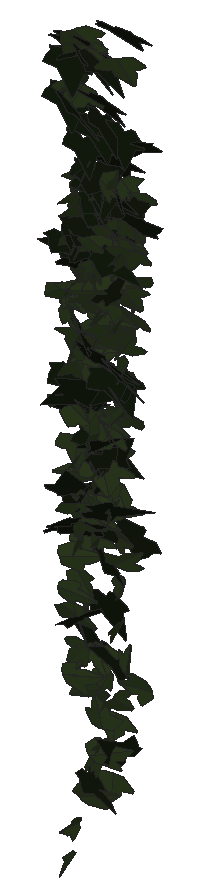
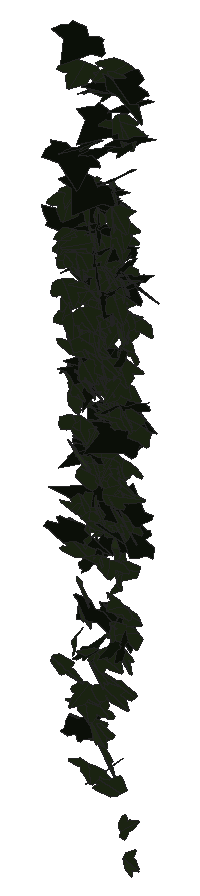
# SketchUp Ruby script. Lengths in millimetres.
U = 1.mm
M = Sketchup.active_model
def pt(a) = Geom::Point3d.new(a.map { |v| v * U })
def face(e, loops, mat)
  f = e.add_face(loops[0].map { |a| pt(a) })
  loops[1..].each { |l| e.add_face(l.map { |a| pt(a) }).erase! }
  f.material = f.back_material = mat if mat
  f
end
# faces: each face lists its corners as indices into pts; further lists are holes
def faces(e, pts, list, mat = nil) = list.each { |f| face(e, (f[0].is_a?(Array) ? f : [f]).map { |l| l.map { |i| pts[i] } }, mat) }
# xy, xz, yz: faces in a plane at the given z, y or x. An outline is a flat list of corners, or four numbers for a rectangle; further outlines are holes
def ring(l) = l.size == 4 ? [[l[0], l[1]], [l[2], l[1]], [l[2], l[3]], [l[0], l[3]]] : l.each_slice(2).to_a
def flat(e, list, mat, &to3) = list.each { |f| face(e, (f[0].is_a?(Array) ? f : [f]).map { |l| ring(l).map { |u, v| to3.(u, v) } }, mat) }
def xy(e, z, list, mat = nil) = flat(e, list, mat) { |x, y| [x, y, z] }
def xz(e, y, list, mat = nil) = flat(e, list, mat) { |x, z| [x, y, z] }
def yz(e, x, list, mat = nil) = flat(e, list, mat) { |y, z| [x, y, z] }
def lines(e, pts, list) = list.each { |a, b| e.add_line(pt(pts[a]), pt(pts[b])) }
# prism: a flat outline (further loops are holes) pulled along v
def prism(e, loops, v, mat = nil)
  f = face(e, loops, mat); d = Geom::Vector3d.new(v.map { |x| x * U })
  f.pushpull(f.normal.samedirection?(d) ? d.length : -d.length)
end
def box(e, o, s, mat = nil) = prism(e, [[o, [o[0] + s[0], o[1], o[2]], [o[0] + s[0], o[1] + s[1], o[2]], [o[0], o[1] + s[1], o[2]]]], [0, 0, s[2]], mat)
def at(x, y, z, deg = 0) = Geom::Transformation.translation(pt([x, y, z])) * Geom::Transformation.rotation(ORIGIN, Z_AXIS, deg.degrees)
def axes(o, x, y, z) = Geom::Transformation.new([*x, 0, *y, 0, *z, 0, *pt(o).to_a, 1])
def part(name) = M.definitions.add(name)
# library, detail: a bought-in or finely detailed component or shape, given as its bounding box
def library(name, o, s) = part(name).tap { |d| box(d.entities, o, s) }
def detail(e, o, s) = box(e.add_group.entities, o, s)
def put(e, d, t, mat = nil) = e.add_instance(d, t).tap { |i| i.material = mat if mat }
def group(e, t, mat = nil) = e.add_group.tap { |g| g.transformation = t; g.material = mat if mat }.entities
root = M.entities
M.materials.add("efeu1").color = [18, 25, 13]
M.materials.add("efeu2").color = [43, 57, 29]
c1 = part("ivyleaf_10")
p = [[0,12.8,-0.8],[-1.5,51.3,-10.9],[-4.9,51,-11.6],[-13.6,26.5,-7.3],[-13.2,15.9,-4.6],[-21.1,19.3,-7.2],
  [-29.5,16.3,-8.3],[-29.2,8.3,-6.2],[-19.7,-9.8,0.5],[-7.6,-13,4],[1,-12.2,5.8],[-0.4,51.1,-11.1],
  [-1.5,51.1,-10.9],[1,-12.4,5.9],[16.9,-12.4,3.5],[35.1,9.1,-5.1],[35,12.9,-6.1],[20.5,16.4,-4.9],
  [15.8,15,-3.8],[15.3,27.6,-7.1],[12.8,31.3,-7.8]]
faces(c1.entities,p,[[0,1,2,3,4,5,6,7,8,9,10],[11,12,0,13,14,15,16,17,18,19,20]],"efeu2")
c2 = part("ivyleaf_9")
p = [[39.1,54.8,31.7],[34.5,51.8,30.2],[-5.3,25.2,17.3],[-17.9,28.3,20.9],[-21.6,21.7,17],[-20.2,4.3,5.3],
  [-22.9,-0.3,2.5],[-17.1,-4,-0.6],[-2,-2.1,-1.2],[-0.7,-15.4,-10.1],[16.6,-22.3,-16.7],[21.1,-15.1,-12.5],
  [32.7,-10.7,-11],[46.1,-1.8,-6.6],[30.8,11.2,3.8]]
faces(c2.entities,p,[[0,1,2,3,4,5,6,7,8,9,10,11,12,13,14]],"efeu1")
put(root,c1,axes([1892.1,998.2,-11],[0.19463,-0.47894,0.44315],[0.19274,-0.43148,-0.48969],[1.2268,0.14377,0.00663]))
put(root,c1,axes([1890.9,1029.1,526.8],[0.05124,0.51211,-0.45605],[-0.09465,-0.45374,-0.51245],[-1.30166,0.05315,0.01931]))
put(root,c2,axes([1892.3,1001.6,639],[1.13233,0.14798,0.48713],[-0.90086,-0.11512,0.61309],[0.3568,-0.76028,0.00198]))
put(root,c1,axes([1879.9,1025.5,845.9],[0.7864,-0.38691,0.46588],[0.74396,-0.26036,-0.56292],[0.88029,0.56568,0.05956]))
put(root,c1,axes([1880.9,995,809.6],[-0.93857,-0.26754,-0.57621],[0.93865,0.29856,-0.56073],[0.76212,-0.6972,-0.019]))
put(root,c1,axes([1898.9,987.2,1003.2],[-0.90015,-0.5253,-0.05863],[0.07791,0.04204,-0.70684],[1.00293,-0.47473,0.00228]))
put(root,c2,axes([1884.6,1004,617.8],[-0.19577,0.57987,0.50112],[0.14823,-0.49509,0.58887],[1.45106,0.12881,0.00746]))
put(root,c1,axes([1893.1,1015.8,1002.9],[0.30987,-0.60948,0.3602],[0.28356,-0.33183,-0.62882],[1.31723,0.21481,0.05063]))
put(root,c2,axes([1923.4,990.5,1092.2],[-1.01779,0.459,0.33561],[-0.52931,0.1907,-0.70398],[-0.9439,-0.60187,0.03289]))
put(root,c1,axes([1884.2,986,1007.1],[-1.08831,-0.15728,-0.38861],[0.79191,-0.13262,-0.5586],[0.09749,-0.67855,0.19926]))
put(root,c1,axes([1901.7,1016.9,1052.5],[-0.44757,-0.68863,0.0359],[-0.02596,-0.03328,-0.72767],[1.31212,-0.23555,-0.00215]))
put(root,c1,axes([1920.8,1003.5,706.2],[-0.09636,0.0198,0.73075],[-1.32281,0.22566,-0.05427],[-0.43108,-0.69688,0.00319]))
put(root,c2,axes([1915.6,986.7,1442.6],[-0.21059,0.78295,0.17358],[-0.28841,0.15166,-0.78065],[-1.49879,-0.13919,0.12583]))
put(root,c1,axes([1914.2,1013,678.4],[-0.07211,-0.00104,0.71493],[-0.69492,-0.61549,-0.02024],[1.16981,-0.36569,0.03204]))
put(root,c1,axes([1877.9,1003.3,959.6],[0.47811,-0.17501,0.64405],[1.05261,-0.33057,-0.30556],[0.71094,0.60715,0.01928]))
put(root,c1,axes([1881.6,1004.1,426.4],[-0.83839,0.06542,-0.49262],[0.93221,-0.054,-0.44517],[-0.15971,-0.65865,-0.01243]))
put(root,c2,axes([1876,992.3,796.5],[0.92716,0.54428,-0.20873],[0.16349,0.20202,0.72728],[1.09732,-0.48998,0.068]))
put(root,c1,axes([1901.7,999.4,47.8],[-0.07165,0.02359,-0.66136],[-0.37794,-0.63231,-0.01125],[-1.20146,0.1975,0.04298]))
put(root,c1,axes([1900.5,997.6,1017.8],[0.06074,-0.68107,-0.2599],[0.06835,0.26131,-0.68033],[1.38569,0.01696,0.04495]))
put(root,c2,axes([1892.4,997.5,1352.9],[-0.51061,-0.73879,-0.08469],[0.06377,0.07793,-0.78599],[1.41385,-0.27033,0.00487]))
put(root,c1,axes([1910.2,1001.1,923.6],[-1.20894,-0.20678,0.21722],[-0.37356,-0.09804,-0.66731],[0.43155,-0.66413,0.03088]))
put(root,c1,axes([1896.5,1007.3,1095],[0.54539,-0.6458,0.24341],[0.22418,-0.21392,-0.70625],[1.29422,0.3092,0.01976]))
put(root,c2,axes([1880,1025.3,410.9],[0.27959,-0.07044,-0.76366],[1.27369,-0.36794,0.16268],[-0.71278,-0.68511,-0.00885]))
put(root,c2,axes([1891.5,994.4,1417.5],[-0.32094,-0.77685,-0.00116],[0.00042,0.00114,-0.79494],[1.47851,-0.16863,-0.00003]))
put(root,c2,axes([1882.8,970.1,588.7],[0.19865,0.77359,-0.37329],[0.09599,0.36987,0.7806],[1.63193,-0.11592,-0.00047]))
put(root,c2,axes([1888.9,1005.2,852],[-0.24132,-0.75891,-0.31784],[0.08183,0.31505,-0.76938],[1.56379,-0.1336,-0.00879]))
put(root,c2,axes([1882.7,996.5,1096.7],[0.13087,-0.62459,-0.43477],[0.27096,0.43939,-0.60871],[1.42278,-0.02623,0.15591]))
put(root,c2,axes([1893.7,996.8,1116],[0.51475,-0.39164,-0.60337],[-0.59231,0.51745,-0.47538],[1.23427,0.41165,0.02351]))
put(root,c1,axes([1907.4,1001.3,1008.6],[-0.60128,-0.56594,0.40793],[-0.0869,-0.43008,-0.63202],[1.32489,-0.28505,0.14368]))
put(root,c2,axes([1888.2,1009.6,1081.7],[0.21259,-0.69257,-0.31477],[-0.0378,0.31538,-0.70096],[1.44735,0.10996,0.02793]))
put(root,c1,axes([1877.9,1005,458.4],[-0.04579,-0.06446,-0.64016],[1.14648,-0.22727,0.00025],[-0.43011,-0.59894,0.06881]))
put(root,c1,axes([1875.1,1007.4,831],[0.66425,0.08698,-0.6989],[1.30234,0.14267,0.35948],[0.31714,-0.76806,-0.01237]))
put(root,c1,axes([1897.5,994.7,1102.9],[-0.49168,-0.51949,-0.50038],[0.53689,0.4164,-0.57795],[1.2634,-0.37912,0.05087]))
put(root,c1,axes([1900.6,1011,891.6],[-0.43543,-0.44557,-0.50735],[0.40774,0.4601,-0.50068],[1.21869,-0.31313,-0.01376]))
put(root,c1,axes([1908.8,1000,1090],[0.39131,-0.68349,-0.24067],[-0.05869,0.24169,-0.71274],[1.37786,0.20441,0.03799]))
put(root,c1,axes([1910.2,1006.8,1212.6],[-0.37225,-0.69304,0.2364],[-0.01059,-0.24328,-0.71779],[1.39357,-0.18697,0.05769]))
put(root,c1,axes([1887.2,1021.1,481.2],[0.86093,-0.12723,0.46148],[0.86001,-0.09607,-0.46943],[0.30069,0.63904,0.02131]))
put(root,c1,axes([1910.2,992.3,1180.1],[-0.38756,-0.71541,-0.11352],[0.02797,0.11382,-0.74364],[1.37832,-0.20347,-0.01683]))
put(root,c1,axes([1909.1,995.3,1381.4],[-0.23018,-0.78256,-0.05289],[0.10289,0.04507,-0.79048],[1.48921,-0.12407,0.04644]))
put(root,c2,axes([1889,1010.7,796.4],[1.33059,0.28438,0.2271],[0.39543,0.09191,-0.75473],[-0.56867,0.72932,0.00656]))
put(root,c1,axes([1912.2,992.3,1158.2],[-0.37361,-0.71421,-0.12632],[0.03883,0.12538,-0.74057],[1.37983,-0.19691,-0.01336]))
put(root,c1,axes([1911.3,992.9,715],[0.12809,-0.66352,-0.22259],[0.00896,0.22404,-0.66642],[1.33194,0.0623,0.02589]))
put(root,c2,axes([1926.3,992.2,838.1],[0.15156,0.15391,-0.78659],[-0.58079,-0.7251,-0.17277],[-1.41053,0.3151,-0.01338]))
put(root,c1,axes([1904.9,1006.3,994],[0.26511,0.60681,0.34219],[-0.06348,0.35438,-0.61484],[-1.32434,0.10449,0.09797]))
put(root,c1,axes([1910.8,990.7,567],[0.17328,-0.46133,-0.60617],[0.0576,0.61219,-0.46137],[1.44863,0.03084,0.09085]))
put(root,c1,axes([1912.9,998.6,572.7],[0.41058,-0.34624,0.53241],[-0.44883,0.47841,0.40669],[-1.12229,-0.318,0.03214]))
put(root,c1,axes([1895.1,1006.7,634.5],[-0.88033,0.32518,-0.48346],[0.7346,-0.29139,-0.56528],[-0.83066,-0.60231,0.01246]))
put(root,c1,axes([1906.3,994.6,876.2],[-0.62994,-0.60809,-0.42999],[0.44353,0.36234,-0.69182],[1.34625,-0.40392,0.02672]))
put(root,c1,axes([1911.9,992.5,1368.5],[1.45429,0.12089,-0.18392],[-0.37101,0.06325,-0.76833],[-0.19447,0.7834,0.09042]))
put(root,c1,axes([1917.3,981.8,914.1],[-0.06072,0.07864,0.80259],[-0.60761,0.73636,-0.08484],[-1.40941,-0.32084,0.002]))
put(root,c2,axes([1890.5,991.8,1344.7],[0.7805,-0.68862,0.00741],[0.02242,-0.00161,-0.80143],[1.31046,0.41016,0.0093]))
put(root,c1,axes([1901,1026.6,432.3],[-0.09377,-0.05383,0.68033],[0.67338,-0.58529,-0.02069],[1.11067,0.35031,0.06998]))
put(root,c1,axes([1886.1,1020.6,837.8],[0.52865,-0.05979,0.6487],[1.23953,0.00986,-0.27797],[0.02748,0.7056,0.05885]))
put(root,c1,axes([1902.1,993.1,736.4],[1.3072,-0.18781,0.22299],[0.4078,-0.06181,-0.71205],[0.37626,0.71948,-0.00296]))
put(root,c2,axes([1885.5,987.4,1455],[1.38474,-0.07712,0.3361],[0.64382,0.00739,-0.73062],[0.12731,0.80143,0.03908]))
put(root,c1,axes([1919.8,987.3,376.6],[0.96125,-0.49047,-0.24955],[-0.30952,0.19055,-0.70369],[1.00056,0.53015,0.02206]))
put(root,c1,axes([1888.9,1003.2,311.2],[0.55941,-0.25205,-0.63911],[1.1567,-0.22872,0.36972],[-0.60964,-0.66524,0.11504]))
put(root,c2,axes([1901.2,1014.7,401.5],[0.87533,-0.56043,-0.25866],[-0.29392,0.20783,-0.7249],[1.13738,0.48502,0.01174]))
put(root,c1,axes([1924,1002.8,639.9],[0.91718,-0.57651,-0.34397],[-0.42094,0.26343,-0.7514],[1.20633,0.53025,-0.00068]))
put(root,c1,axes([1920.5,1000,1035.6],[0.18194,-0.43647,-0.55522],[-0.08957,0.5551,-0.44448],[1.34114,0.09629,0.04564]))
put(root,c2,axes([1926.6,977.9,439.8],[0.09141,0.80891,-0.11699],[-0.01363,-0.11677,-0.81033],[-1.55547,0.04856,0.00023]))
put(root,c1,axes([1930.1,992,1042.8],[-1.08717,0.24738,0.35267],[-0.65261,0.09344,-0.62094],[-0.49627,-0.6648,0.04395]))
put(root,c1,axes([1936.4,1003.7,301.4],[-0.82061,-0.12625,0.49892],[-0.8843,-0.18438,-0.4482],[0.42116,-0.63312,0.03104]))
put(root,c1,axes([1912.4,988.8,624.2],[-1.18125,-0.27224,-0.27051],[0.48408,0.09338,-0.67757],[0.54698,-0.67058,0.01547]))
put(root,c1,axes([1912.9,1003.7,799.4],[-0.41144,0.67613,-0.22758],[0.13256,-0.21666,-0.70985],[-1.35125,-0.22713,-0.00034]))
put(root,c1,axes([1895.9,987.3,532.2],[0.30838,-0.02507,-0.72057],[1.22012,0.34296,0.13223],[0.62792,-0.6541,0.09695]))
put(root,c2,axes([1904.8,1000,1114.9],[0.66517,-0.65413,-0.27341],[-0.25101,0.23952,-0.74164],[1.32576,0.37354,-0.00324]))
put(root,c1,axes([1924,1010.1,1106.8],[0.75239,0.47162,-0.37486],[-0.53552,-0.25191,-0.61368],[-1.01384,0.48306,0.04596]))
put(root,c1,axes([1912.2,1022.7,558],[1.30456,0.17596,0.05789],[0.10704,0.01372,-0.70768],[-0.3359,0.68776,-0.00069]))
put(root,c1,axes([1922.5,996.3,1216.1],[0.13534,-0.69905,-0.33591],[0.05284,0.3394,-0.70043],[1.47511,0.05198,0.05591]))
put(root,c2,axes([1916.9,989.5,1065.2],[1.13263,0.55736,-0.0919],[-0.13999,-0.05589,-0.81531],[-1.06593,0.59957,0.00943]))
put(root,c2,axes([1908.4,1009,925.5],[0.032,-0.46123,0.64664],[0.06277,-0.64582,-0.4615],[1.51037,0.03661,0.00548]))
put(root,c1,axes([1918.7,1016.7,1139.9],[-0.04191,0.72956,0.00263],[-0.07678,0.00141,-0.72878],[-1.38639,-0.02213,0.04028]))
put(root,c2,axes([1910.9,980.6,591.9],[1.11611,0.51336,0.23414],[0.33039,0.15716,-0.77938],[-1.02176,0.61158,0.00374]))
put(root,c1,axes([1920.7,997.3,995.2],[0.52872,-0.63305,0.29001],[-0.20635,0.26911,0.69127],[-1.30907,-0.2981,0.00817]))
put(root,c2,axes([1912.5,996.4,1137.8],[-0.05122,-0.58734,-0.53182],[-0.02432,0.53238,-0.58731],[1.50778,-0.01136,-0.02754]))
put(root,c2,axes([1914.5,1000.2,1275.7],[-0.07729,-0.7675,0.06321],[-0.03723,-0.06225,-0.76841],[1.46518,-0.04207,-0.01619]))
put(root,c1,axes([1932.1,1012.3,367.2],[-0.30963,-0.56482,0.49986],[-0.13152,-0.49805,-0.58526],[1.42944,-0.16817,0.05443]))
put(root,c1,axes([1917.7,1022.2,1093.1],[-1.25445,0.00623,-0.29854],[0.54977,-0.16994,-0.64132],[-0.14394,-0.70334,0.15231]))
put(root,c1,axes([1902.8,1012.9,1083],[-0.319,0.08875,-0.75291],[1.07714,-0.4984,-0.18474],[-0.96001,-0.5887,0.0429]))
put(root,c1,axes([1922.3,1017.4,1105.7],[0.93783,-0.51482,0.20548],[0.25609,-0.15562,-0.71257],[1.02341,0.51071,-0.00999]))
put(root,c1,axes([1933.4,1007.6,882.3],[0.71121,-0.61341,-0.26092],[-0.25547,0.22375,-0.71827],[1.24267,0.39707,0.00167]))
put(root,c1,axes([1929.6,989.2,1242.6],[0.46693,-0.68859,-0.20788],[0.01124,0.22156,-0.72693],[1.36889,0.23306,0.07688]))
put(root,c1,axes([1906.2,993.8,790.4],[0.94969,0.19908,0.54455],[0.96194,0.20268,-0.53724],[-0.5407,0.71025,0.00067]))
put(root,c1,axes([1934,1013.7,930.1],[0.26379,-0.62847,-0.31118],[-0.08545,0.3086,-0.64325],[1.33196,0.14426,0.02036]))
put(root,c1,axes([1926.3,1024.8,765.1],[-1.25412,0.03998,0.2448],[0.43361,-0.17716,0.64222],[0.18664,0.68027,0.15286]))
put(root,c1,axes([1918.6,983,1474.6],[-1.00542,-0.33645,-0.52555],[0.89375,0.23911,-0.62512],[0.78211,-0.70577,0.03875]))
put(root,c1,axes([1952.3,996.7,1023.7],[-0.38752,-0.13137,0.67808],[-0.90299,-0.48713,-0.23685],[0.95528,-0.51376,0.05119]))
put(root,c1,axes([1915.7,988.3,1450.2],[-1.11537,-0.11385,-0.54676],[1.04789,0.01498,-0.59328],[0.17805,-0.80136,0.06659]))
put(root,c1,axes([1924.9,1022.3,562.4],[-0.20566,0.12708,0.71764],[0.61357,-0.64231,0.16228],[1.24397,0.33782,0.0386]))
put(root,c1,axes([1950.7,1014.1,616.5],[0.44163,0.33033,0.58383],[-0.80214,-0.40881,0.39882],[0.99321,-0.47705,0.0625]))
put(root,c1,axes([1911.8,1022,919.4],[0.67147,-0.17142,-0.59477],[0.99413,-0.28486,0.39195],[-0.63205,-0.63015,-0.01539]))
put(root,c1,axes([1942.6,999.7,180],[0.65294,-0.54592,-0.33052],[-0.34274,0.27718,-0.64476],[1.16522,0.38744,-0.00444]))
put(root,c1,axes([1936.4,989,730.3],[-0.45843,0.69085,0.26597],[-0.17315,0.24995,-0.73163],[-1.39823,-0.25746,0.0034]))
put(root,c1,axes([1937.9,1005.8,881.8],[1.50158,0.03802,-0.10984],[-0.20874,-0.006,-0.78989],[-0.07325,0.79656,-0.00071]))
put(root,c1,axes([1942.1,986.8,1011.5],[-0.75915,-0.57839,-0.13095],[0.11239,0.11829,-0.70236],[1.12303,-0.40282,-0.01823]))
put(root,c1,axes([1944.6,1001.8,1065.3],[-0.29286,-0.65037,0.30454],[-0.04578,-0.30661,-0.66695],[1.36601,-0.14971,0.04294]))
put(root,c1,axes([1942.5,1004.5,981.1],[0.11031,-0.52571,-0.47393],[0.02626,0.47626,-0.52661],[1.34682,0.03377,0.04909]))
put(root,c1,axes([1964.9,1009.4,703.1],[-0.48681,-0.2451,0.72492],[-1.0387,-0.47734,-0.35396],[1.02086,-0.60256,-0.01446]))
put(root,c1,axes([1920,1001.7,895.2],[0.56382,-0.02612,-0.6077],[1.08653,0.24521,0.26777],[0.3995,-0.63003,0.12941]))
put(root,c1,axes([1933.6,980,610.4],[-0.35906,-0.40508,-0.63403],[0.65242,0.5356,-0.44419],[1.27468,-0.38824,0.04875]))
put(root,c2,axes([1923.2,991.6,1439.3],[0.71872,-0.70336,0.07002],[0.03514,-0.06955,-0.79815],[1.34479,0.37773,-0.01657]))
put(root,c1,axes([1935,1024.1,653.1],[0.6693,-0.49671,0.35568],[0.46474,-0.2619,-0.60719],[1.06579,0.42613,0.04141]))
put(root,c2,axes([1959.6,1009.2,1119.7],[0.19164,-0.05214,-0.7918],[-1.38216,0.31559,-0.11314],[0.60859,0.73313,-0.00761]))
put(root,c1,axes([1927,992.9,111.2],[-0.65757,-0.18373,0.5424],[0.89402,0.2714,0.39116],[-0.62339,0.58302,-0.01116]))
put(root,c2,axes([1932.5,993.7,150.5],[0.51932,-0.65451,-0.29958],[-0.20542,0.27956,-0.70908],[1.35447,0.29335,0.00732]))
put(root,c1,axes([1953.2,999.7,1144.1],[-1.34632,-0.16324,0.07957],[-0.14442,-0.02501,-0.72595],[0.314,-0.71142,0.00727]))
put(root,c1,axes([1950.1,1008.6,972.4],[-0.16452,-0.67752,-0.19305],[0.03216,0.19245,-0.68297],[1.34039,-0.08778,-0.00731]))
put(root,c2,axes([1939.1,998.6,1233.8],[-0.31276,-0.74586,-0.09981],[0.04515,0.09697,-0.76374],[1.43146,-0.16602,0.00228]))
put(root,c1,axes([1933.3,996.5,615],[-0.76551,-0.21698,-0.51948],[0.92076,0.19327,-0.45532],[0.54792,-0.62793,0.03937]))
put(root,c1,axes([1954.1,1007.4,1089],[0.48801,-0.5036,-0.45479],[-0.23543,0.44334,-0.56066],[1.2698,0.27574,0.07083]))
put(root,c2,axes([1934.6,1003.9,1179.3],[0.28195,-0.71982,-0.27685],[-0.06524,0.27549,-0.73461],[1.46634,0.15066,0.02055]))
put(root,c1,axes([1940.2,1005.7,368.8],[0.94003,0.50186,0.11537],[0.15245,0.08304,-0.70415],[-0.96813,0.50037,0.00114]))
put(root,c1,axes([1955.6,980.7,1072.5],[-0.30816,0.46259,0.62237],[-0.53006,0.55868,-0.48771],[-1.37738,-0.31849,0.04845]))
put(root,c1,axes([1961.7,1026.7,962.9],[0.60939,0.39936,-0.48285],[-0.89335,-0.20633,-0.48192],[-0.79,0.54138,0.17251]))
put(root,c1,axes([1944,999.1,729.5],[-1.4469,-0.05515,-0.26231],[0.50043,-0.00024,-0.76203],[0.09907,-0.80423,0.01821]))
put(root,c2,axes([1945.3,1005.4,1154.6],[-0.0141,0.41853,0.67624],[-0.38344,-0.6552,0.4033],[1.4642,-0.16755,0.11213]))
put(root,c1,axes([1930.7,1009.2,785.4],[-0.81337,0.04164,-0.59608],[1.13479,-0.0183,-0.42877],[-0.07451,-0.73323,-0.02315]))
put(root,c1,axes([1949.6,1010.7,795.4],[-1.21488,-0.27201,-0.18089],[0.31324,0.07519,-0.69386],[0.53704,-0.65919,-0.0045]))
put(root,c2,axes([1945.2,1006.6,752.9],[-0.5645,-0.7166,-0.13537],[0.1152,0.12144,-0.7755],[1.38316,-0.30258,0.00934]))
put(root,c1,axes([1957.1,993.7,255.3],[1.28331,-0.18321,0.26968],[-0.49805,0.06536,0.69872],[-0.37007,-0.72327,-0.00517]))
put(root,c1,axes([1950.8,991.3,695.5],[0.5294,-0.66408,0.30344],[-0.17642,0.28996,0.71957],[-1.37832,-0.29218,0.02444]))
put(root,c1,axes([1969.6,1012.3,625.4],[0.52137,0.3777,0.53924],[-0.79831,-0.35004,0.45827],[0.96575,-0.49325,0.0877]))
put(root,c1,axes([1955.1,1028.8,914.7],[-0.26508,-0.63759,0.28466],[0.13215,-0.30148,-0.64128],[1.32232,-0.09769,0.12115]))
put(root,c1,axes([1952.2,974.1,776.5],[-0.00441,-0.30338,-0.83146],[0.30271,0.81778,-0.29883],[1.65706,-0.1502,0.05238]))
put(root,c1,axes([1956.9,1011.3,1168.9],[0.18485,-0.72908,-0.13783],[0.00012,0.13901,-0.7353],[1.41216,0.09542,0.0181]))
put(root,c1,axes([1953.9,993.2,702.9],[0.25345,-0.67555,0.22901],[0.18599,-0.21349,-0.6866],[1.34478,0.15685,0.0518]))
put(root,c2,axes([1940.8,987.5,1368.8],[1.54997,0.01201,-0.13431],[-0.25576,0.0046,-0.81446],[-0.02114,0.82539,0.0065]))
put(root,c1,axes([1960.7,1028.6,1015.5],[-0.50901,-0.59595,0.26997],[-0.0398,-0.28371,-0.64702],[1.24453,-0.25282,0.08972]))
put(root,c1,axes([1958.2,999.4,216.9],[0.16325,-0.7222,0.17778],[0.02918,-0.1772,-0.72725],[1.41521,0.08696,-0.00551]))
put(root,c1,axes([1955.2,1005.3,333.2],[0.95709,-0.50567,0.00594],[0.00806,-0.00417,-0.71316],[0.96242,0.5029,0.00006]))
put(root,c1,axes([1960.7,1004.1,953.9],[-0.84146,-0.57436,-0.02969],[0.03684,0.02257,-0.72482],[1.09396,-0.44255,0.00157]))
put(root,c2,axes([1927.4,985.3,912],[1.34648,-0.2876,0.34109],[0.59984,-0.13042,-0.7637],[0.601,0.77451,-0.00194]))
put(root,c1,axes([1944.8,988.9,1110.2],[-1.00503,-0.2354,-0.43997],[0.85826,0.04907,-0.56752],[0.40651,-0.68558,0.11044]))
put(root,c2,axes([1949.8,1013.4,1252.9],[1.43791,0.27204,-0.16937],[-0.30901,-0.049,-0.80296],[-0.52581,0.77272,0.00871]))
put(root,c2,axes([1949.3,998,1317.3],[-0.25148,-0.75978,-0.12015],[0.02036,0.12009,-0.77112],[1.46383,-0.1322,-0.00992]))
put(root,c2,axes([1951.5,998.2,1217.4],[-0.57734,-0.60901,-0.34469],[0.30012,0.30652,-0.68037],[1.29758,-0.34187,0.004]))
put(root,c2,axes([1944.2,1021.6,457.9],[-0.65801,-0.04026,-0.71456],[1.34681,0.0994,-0.348],[0.20361,-0.78756,-0.00739]))
put(root,c2,axes([1948.5,1004.3,778.4],[-0.00529,-0.18732,0.78527],[0.04262,-0.78499,-0.18718],[1.53586,0.02114,0.0079]))
put(root,c2,axes([1957,996,1217.2],[-0.82081,-0.60944,-0.25471],[0.24045,0.22247,-0.74622],[1.23391,-0.44876,-0.02402]))
put(root,c1,axes([1965.4,999.2,1194.7],[-0.27743,-0.71295,0.21921],[0.01573,-0.22488,-0.72592],[1.41948,-0.13685,0.05089]))
put(root,c2,axes([1944.5,994.6,1438.7],[0.40087,-0.73632,-0.18532],[0.07171,0.20222,-0.76064],[1.4433,0.19447,0.08926]))
put(root,c2,axes([1972.3,980.2,765],[0.30643,0.74686,-0.28948],[-0.11546,-0.28305,-0.76402],[-1.52008,0.17206,-0.00033]))
put(root,c2,axes([1947.2,1004.7,782.2],[0.04125,-0.38397,0.73859],[0.25587,-0.72753,-0.38217],[1.5635,0.12919,0.04306]))
put(root,c2,axes([1949.9,1002.2,1167.7],[0.03655,-0.51694,-0.59518],[0.21538,0.591,-0.50965],[1.48481,-0.073,0.08858]))
put(root,c2,axes([1971.5,1013.8,357.7],[0.41475,-0.72711,-0.12893],[0.0729,-0.12311,0.75907],[-1.40353,-0.22126,0.00133]))
put(root,c1,axes([1986.4,981.8,1015.5],[0.59665,-0.11368,-0.65168],[-0.98158,0.4096,-0.31956],[0.78842,0.59598,0.09532]))
put(root,c1,axes([1969.4,992.1,776.7],[1.3353,-0.08805,-0.14276],[-0.26611,0.03209,-0.70697],[0.17631,0.71527,0.01415]))
put(root,c1,axes([1962.4,1009.5,147.7],[1.34722,-0.0304,0.07421],[0.14187,0.0062,-0.70846],[0.05631,0.71172,0.00934]))
put(root,c2,axes([1951.6,987.1,1236.9],[0.16279,-0.38612,-0.69976],[0.29489,0.69842,-0.36644],[1.49223,-0.0959,0.14876]))
put(root,c1,axes([1970.8,1023.8,493.1],[0.69327,-0.60825,0.00946],[0.00921,-0.00812,-0.70898],[1.15772,0.3643,-0.00002]))
put(root,c2,axes([1957.3,1008.1,535.6],[0.8287,-0.43084,-0.46948],[0.64303,-0.32601,0.61253],[-1.02823,-0.55112,0.00468]))
put(root,c2,axes([1956.7,997.2,1330.6],[0.19777,-0.76514,0.1623],[0.02021,-0.16233,-0.77209],[1.48848,0.10386,-0.01108]))
put(root,c1,axes([1944.1,1000.6,981.5],[0.27501,0.07148,0.74661],[1.23929,0.36535,-0.161],[-0.70835,0.66695,0.00818]))
put(root,c2,axes([1980.8,999.2,1188.4],[0.25345,-0.43472,0.65491],[-0.11063,0.65698,0.44792],[-1.49194,-0.12257,0.07804]))
put(root,c1,axes([1965.8,1020.3,630.5],[1.39952,-0.13555,-0.05695],[0.10689,-0.00943,0.74774],[-0.2586,-0.73749,0.0009]))
put(root,c1,axes([1987.5,1020.7,798.4],[-1.11529,-0.11328,0.30476],[-0.57658,-0.0378,-0.59658],[0.22464,-0.65943,-0.01815]))
put(root,c1,axes([1964.2,984,717.2],[1.28781,0.5304,0.11601],[0.1672,0.07596,-0.85974],[-1.0197,0.68231,0.00554]))
put(root,c1,axes([1955.7,1010.8,1144.8],[0.49913,0.22393,0.65302],[0.7606,0.52036,-0.33894],[-1.07133,0.47376,0.06361]))
put(root,c1,axes([1971,1009.5,292.3],[-0.5166,-0.47357,-0.53168],[0.47965,0.46826,-0.54575],[1.26736,-0.37026,-0.01018]))
put(root,c1,axes([1974.7,1003.3,643.1],[0.28232,-0.6526,0.26133],[0.20062,-0.24342,-0.6677],[1.32278,0.1762,0.04549]))
put(root,c1,axes([1971,1006.9,260.2],[1.32148,0.04049,0.03455],[0.06566,0.0019,-0.69553],[-0.07715,0.6952,-0.00011]))
put(root,c1,axes([1980.4,1009.6,972.3],[0.17502,-0.68411,-0.08529],[-0.04235,0.08306,-0.69018],[1.3114,0.09398,-0.0109]))
put(root,c1,axes([1983.6,1014.2,1108.7],[-0.85522,-0.52397,0.23775],[-0.07989,-0.27101,-0.6766],[1.09217,-0.43012,0.13668]))
put(root,c1,axes([1978.4,1019.7,1111.5],[1.20484,0.32594,-0.16511],[-0.33023,-0.0225,-0.70968],[-0.61197,0.65385,0.05789]))
put(root,c1,axes([1987.1,1001.4,1153.5],[-1.22986,0.29281,0.17903],[-0.40265,-0.03933,-0.69933],[-0.51431,-0.66939,0.1194]))
put(root,c1,axes([1967.8,1004.7,858],[1.02723,-0.62544,-0.17542],[0.21181,-0.13566,0.82612],[-1.21799,-0.55108,-0.00428]))
put(root,c2,axes([1980,981.1,864.5],[0.98783,-0.11952,-0.56893],[-1.01116,0.2121,-0.52926],[0.44917,0.74034,0.05978]))
put(root,c1,axes([1971.4,998.6,1048.6],[0.84063,0.56045,0.16679],[0.13208,0.1573,-0.71236],[-1.10501,0.44516,0.04174]))
put(root,c1,axes([1979.3,975.2,1231.5],[-0.20418,0.60223,0.49338],[-0.16739,0.48548,-0.61171],[-1.4722,-0.13872,0.00112]))
put(root,c2,axes([1967.5,987.2,736.8],[0.09441,-0.18551,-0.74559],[0.04237,0.74717,-0.18442],[1.46165,-0.00968,0.0535]))
put(root,c1,axes([1964.1,1022.8,727.2],[0.21686,-0.43975,-0.5067],[0.68215,-0.39457,0.42303],[-1.07939,-0.33771,0.16555]))
put(root,c2,axes([1958.2,975.3,640.3],[0.46293,0.53868,-0.57318],[0.43874,0.52479,0.59104],[1.43129,-0.3351,0.00422]))
put(root,c1,axes([2002,1008.2,1106.9],[-1.0264,-0.1143,0.4786],[-0.87186,-0.14255,-0.55026],[0.34183,-0.70681,0.03358]))
put(root,c1,axes([1982.7,1020.4,1110.5],[0.88941,-0.55935,-0.13133],[-0.02666,0.15814,-0.7234],[1.09318,0.45895,0.0892]))
put(root,c2,axes([1968.6,1002,733.2],[-0.43049,0.33505,0.65354],[0.50405,-0.60061,0.39958],[1.3037,0.34285,0.06131]))
put(root,c1,axes([1981.6,992.5,1229.5],[-0.04758,-0.68682,-0.38033],[0.24839,0.37159,-0.67962],[1.47339,-0.08482,0.10229]))
put(root,c1,axes([1957,986.5,200.7],[0.80398,-0.04589,-0.61922],[1.18089,0.00287,0.42308],[-0.0447,-0.74959,0.03953]))
put(root,c2,axes([1997,997.6,873],[-1.3658,0.32819,-0.21715],[0.37813,-0.08768,-0.78912],[-0.6465,-0.74463,-0.00279]))
put(root,c2,axes([1992.1,1007,200.7],[0.28517,0.1017,0.75128],[-1.16739,-0.43382,0.18106],[0.84801,-0.63141,-0.00339]))
put(root,c2,axes([1980.1,972.7,1028],[-0.6226,0.74766,-0.00718],[-0.01476,0.00444,0.81608],[1.42294,0.32718,0.00533]))
put(root,c1,axes([1994,1015.7,1102.3],[-1.07261,-0.39166,0.28473],[-0.26761,-0.28572,-0.67133],[0.88185,-0.56308,0.1426]))
put(root,c1,axes([1986.6,999.5,437.5],[0.22531,-0.70682,0.06284],[0.01956,-0.062,-0.71666],[1.35038,0.11883,-0.0001]))
put(root,c2,axes([2013.2,1021,592.7],[-0.1537,-0.06061,-0.80323],[-1.24568,-0.4656,0.10094],[-0.8936,0.65947,-0.00256]))
put(root,c1,axes([1989.8,1001.7,1099.2],[0.141,-0.75275,-0.07547],[-0.02943,0.07431,-0.75634],[1.43951,0.07525,-0.00807]))
put(root,c1,axes([1975.4,1001.4,1158.2],[0.02369,-0.2504,-0.73782],[0.72886,0.64459,-0.21229],[1.29139,-0.35921,0.13336]))
put(root,c2,axes([1971.6,982.8,1097.8],[0.50036,-0.48913,-0.52554],[-0.04186,0.55392,-0.52654],[1.36574,0.19617,0.1764]))
put(root,c1,axes([1982.1,1006.2,927.9],[-1.31138,-0.3434,0.20197],[0.34521,0.08886,0.76987],[-0.67509,0.71251,0.00133]))
put(root,c1,axes([1968.5,1015.9,579],[-0.41588,0.12823,0.66954],[1.12913,-0.31054,0.2531],[0.63905,0.63214,-0.01148]))
put(root,c1,axes([1999.2,1013.9,985],[-1.27235,0.11193,0.15883],[-0.30095,0.01729,-0.67778],[-0.21489,-0.68692,0.00882]))
put(root,c2,axes([1974.9,984.8,905.5],[1.20455,-0.50166,-0.11268],[-0.16917,0.06926,-0.80761],[0.96382,0.63912,-0.00093]))
put(root,c2,axes([2005.9,993.4,1185.2],[-1.40388,-0.08579,0.17903],[0.35144,-0.04359,0.73995],[-0.13871,0.7578,0.06283]))
put(root,c2,axes([2000.8,1006.1,1296.4],[0.74577,0.65063,-0.26938],[-0.31088,-0.21589,-0.75904],[-1.30367,0.42368,0.0269]))
put(root,c1,axes([1997.2,1000.7,1092],[0.18418,-0.63529,0.37446],[0.08295,-0.37208,-0.64252],[1.40104,0.10554,-0.01119]))
put(root,c2,axes([1988.4,1007.5,1311],[-0.30518,-0.75,0.06774],[0.00337,-0.06963,-0.76678],[1.43321,-0.15954,0.01623]))
put(root,c2,axes([1984.1,990.2,882.8],[-0.51012,-0.61427,-0.44928],[0.44449,0.38695,-0.66838],[1.37851,-0.35208,0.04926]))
put(root,c1,axes([1986.9,1001.4,544.4],[-0.7291,-0.40564,0.35463],[0.48667,0.24613,0.55776],[-0.9026,0.46037,0.01427]))
put(root,c1,axes([1985.7,1022.8,866.6],[0.91687,-0.33325,0.38155],[0.59857,-0.21603,-0.58578],[0.75584,0.57532,0.00105]))
put(root,c1,axes([1996.1,1027.1,1019.6],[-0.28355,0.5728,-0.39445],[-0.07909,-0.41001,-0.5797],[-1.32127,-0.09838,0.11935]))
put(root,c2,axes([1990.4,984.3,1508.6],[1.45836,0.21565,-0.16634],[-0.36131,0.06679,-0.78793],[-0.37165,0.78127,0.11327]))
put(root,c1,axes([2006.5,1020.9,1047.9],[-0.75353,-0.59563,0.10264],[-0.12174,-0.08072,-0.71517],[1.14385,-0.40097,-0.0085]))
put(root,c1,axes([2001.4,1002,832.4],[0.04593,-0.51784,0.66794],[0.12206,-0.66516,-0.518],[1.60387,0.06545,0.02029]))
put(root,c1,axes([2004,992.4,369.1],[0.04723,0.30738,-0.70426],[-0.02447,0.70469,0.30711],[1.46224,0.00187,0.02789]))
put(root,c1,axes([2003.7,988.3,908.1],[0.5412,-0.74754,-0.14267],[-0.06309,0.13999,-0.79959],[1.44703,0.28569,0.01849]))
put(root,c1,axes([2008.1,994.8,1108.1],[-1.35321,-0.21664,0.04594],[-0.08164,-0.01685,-0.74328],[0.41349,-0.7123,0.00361]))
put(root,c1,axes([1998.1,987.4,1448.4],[-1.17588,-0.4569,-0.25888],[0.48779,0.08653,-0.76442],[0.87234,-0.66428,0.07849]))
put(root,c1,axes([2004.2,1002.9,950],[0.09998,-0.60983,0.38108],[0.06136,-0.37972,-0.61209],[1.36723,0.06164,-0.0004]))
put(root,c1,axes([1999,1001.2,1031.6],[-1.00332,-0.47,-0.32575],[0.45839,0.21935,-0.70626],[0.9871,-0.57958,-0.00313]))
put(root,c1,axes([1999.4,1000,1225.6],[0.22387,0.65612,0.32799],[-0.05514,0.33608,-0.66191],[-1.39498,0.09201,0.0788]))
put(root,c1,axes([2023.6,1015,326.9],[0.45603,-0.16729,-0.63413],[-1.00187,0.3536,-0.29219],[0.74443,0.57836,-0.00478]))
put(root,c1,axes([2001,1014.8,1144.5],[-0.59707,-0.58889,-0.31315],[0.40531,0.2395,-0.66374],[1.20293,-0.37299,0.06821]))
put(root,c1,axes([2007,1007.5,1203.2],[-1.21397,-0.39899,-0.13729],[0.26949,0.03201,-0.75088],[0.75648,-0.65168,0.04718]))
put(root,c2,axes([2007.8,1007,1152.2],[1.25573,-0.17942,0.43297],[-0.7497,0.1928,0.68018],[-0.48329,-0.76526,0.06985]))
